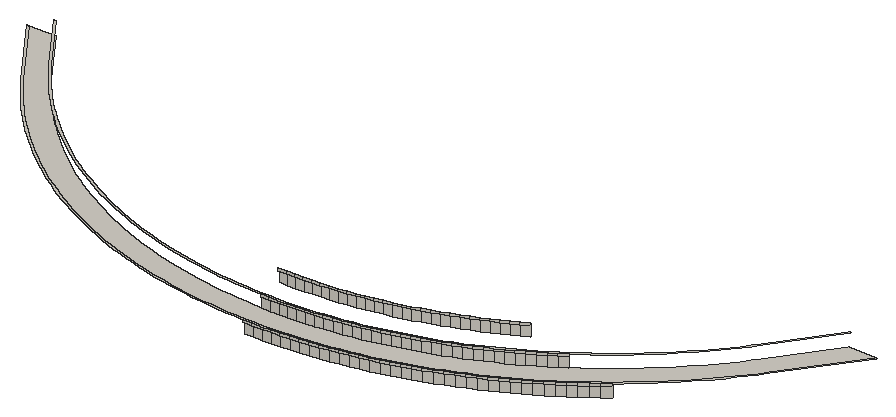
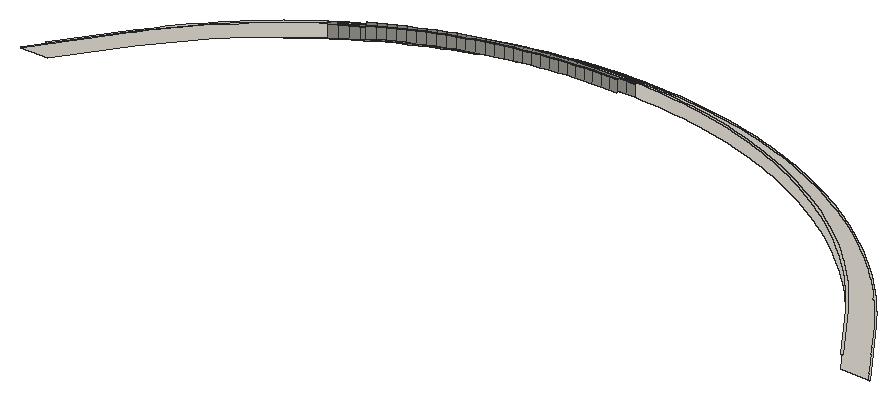
# SketchUp Ruby script. Lengths in inches.
U = 1.inch
M = Sketchup.active_model
def pt(a) = Geom::Point3d.new(a.map { |v| v * U })
def face(e, loops, mat)
  f = e.add_face(loops[0].map { |a| pt(a) })
  loops[1..].each { |l| e.add_face(l.map { |a| pt(a) }).erase! }
  f.material = f.back_material = mat if mat
  f
end
# faces: each face lists its corners as indices into pts; further lists are holes
def faces(e, pts, list, mat = nil) = list.each { |f| face(e, (f[0].is_a?(Array) ? f : [f]).map { |l| l.map { |i| pts[i] } }, mat) }
# xy, xz, yz: faces in a plane at the given z, y or x. An outline is a flat list of corners, or four numbers for a rectangle; further outlines are holes
def ring(l) = l.size == 4 ? [[l[0], l[1]], [l[2], l[1]], [l[2], l[3]], [l[0], l[3]]] : l.each_slice(2).to_a
def flat(e, list, mat, &to3) = list.each { |f| face(e, (f[0].is_a?(Array) ? f : [f]).map { |l| ring(l).map { |u, v| to3.(u, v) } }, mat) }
def xy(e, z, list, mat = nil) = flat(e, list, mat) { |x, y| [x, y, z] }
def xz(e, y, list, mat = nil) = flat(e, list, mat) { |x, z| [x, y, z] }
def yz(e, x, list, mat = nil) = flat(e, list, mat) { |y, z| [x, y, z] }
def lines(e, pts, list) = list.each { |a, b| e.add_line(pt(pts[a]), pt(pts[b])) }
# prism: a flat outline (further loops are holes) pulled along v
def prism(e, loops, v, mat = nil)
  f = face(e, loops, mat); d = Geom::Vector3d.new(v.map { |x| x * U })
  f.pushpull(f.normal.samedirection?(d) ? d.length : -d.length)
end
def box(e, o, s, mat = nil) = prism(e, [[o, [o[0] + s[0], o[1], o[2]], [o[0] + s[0], o[1] + s[1], o[2]], [o[0], o[1] + s[1], o[2]]]], [0, 0, s[2]], mat)
def at(x, y, z, deg = 0) = Geom::Transformation.translation(pt([x, y, z])) * Geom::Transformation.rotation(ORIGIN, Z_AXIS, deg.degrees)
def axes(o, x, y, z) = Geom::Transformation.new([*x, 0, *y, 0, *z, 0, *pt(o).to_a, 1])
def part(name) = M.definitions.add(name)
# library, detail: a bought-in or finely detailed component or shape, given as its bounding box
def library(name, o, s) = part(name).tap { |d| box(d.entities, o, s) }
def detail(e, o, s) = box(e.add_group.entities, o, s)
def put(e, d, t, mat = nil) = e.add_instance(d, t).tap { |i| i.material = mat if mat }
def group(e, t, mat = nil) = e.add_group.tap { |g| g.transformation = t; g.material = mat if mat }.entities
root = M.entities
M.materials.add("Arta-Ceramic-Moonstone-White-24x24-4K").color = [209, 205, 196]
xy(root,6,[[1024.28,78.45,1028.24,78.49,1032.2,78.6,1036.16,78.79,1040.11,79.06,1044.06,79.4,1048,79.82,1051.93,80.31,1055.85,80.88,1059.76,81.52,1063.65,82.24,1067.53,83.03,1071.4,83.9,1075.25,84.84,1079.08,85.85,1082.89,86.94,1086.67,88.1,1090.4375,89.34,1094.18,90.64,1097.89,92.02,1101.58,93.47,1105.24,94.99,1108.87,96.57,1112.47,98.23,1116.03,99.96,1119.5625,101.75,1123.0625,103.61,1126.52,105.54,1129.94,107.54,1133.33,109.6,1136.67,111.72,1139.97,113.91,1143.23,116.16,1146.45,118.47,1149.62,120.85,1152.74,123.28,1155.82,125.78,1158.85,128.33,1161.83,130.94,1164.76,133.61,1167.64,136.33,1170.46,139.11,1173.23,141.94,1175.95,144.82,1178.61,147.76,1181.21,150.75,1183.76,153.78,1186.24,156.87,1188.67,160,1191.04,163.17,1213.38,194.4,1212.72,194.875,1190.38,163.65,1188.02,160.49,1185.6,157.37,1183.13,154.3,1180.59,151.27,1178,148.3,1175.35,145.375,1172.65,142.5,1169.89,139.68,1167.07,136.92,1164.21,134.2,1161.29,131.55,1158.32,128.95,1155.3,126.4,1152.24,123.92,1149.125,121.49,1145.97,119.13,1142.76,116.82,1139.52,114.58,1136.23,112.4,1132.9,110.29,1129.53,108.24,1126.12,106.25,1122.67,104.33,1119.1875,102.47,1115.67,100.6875,1112.12,98.97,1108.54,97.32,1104.92,95.73,1101.28,94.22,1097.6,92.78,1093.9,91.41,1090.18,90.11,1086.43,88.88,1082.66,87.72,1078.86,86.64,1075.05,85.63,1071.21,84.69,1067.36,83.83,1063.5,83.04,1059.62,82.32,1055.72,81.68,1051.82,81.12,1047.9,80.625,1043.98,80.21,1040.05,79.87,1036.11,79.6,1032.17,79.42,1028.23,79.3,1024.28,79.26,1020.34,79.3,1016.39,79.42,1012.45,79.6,1008.51,79.87,1004.58,80.21,1000.66,80.625,996.74,81.12,992.84,81.68,988.94,82.32,985.0625,83.04,981.2,83.83,977.35,84.69,973.51,85.63,969.7,86.64,965.91,87.72,962.13,88.88,958.38,90.11,954.66,91.41,950.96,92.78,947.29,94.22,943.64,95.73,940.03,97.32,936.44,98.97,932.89,100.6875,929.37,102.47,925.89,104.33,922.44,106.25,919.03,108.24,915.66,110.29,912.33,112.4,909.04,114.58,905.8,116.82,902.59,119.13,899.44,121.49,896.32,123.92,893.26,126.4,890.24,128.95,887.27,131.55,884.36,134.2,881.49,136.92,878.68,139.68,875.92,142.5,873.21,145.375,870.5625,148.3,867.97,151.27,865.43,154.3,862.96,157.37,860.54,160.49,858.18,163.65,835.84,194.875,834.84,194.875,857.53,163.17,859.89,160,862.32,156.87,864.81,153.78,867.35,150.75,869.95,147.76,872.61,144.82,875.33,141.94,878.1,139.11,880.92,136.33,883.8,133.61,886.73,130.94,889.71,128.33,892.74,125.78,895.82,123.28,898.94,120.85,902.11,118.47,905.33,116.16,908.59,113.91,911.89,111.72,915.23,109.6,918.62,107.54,922.04,105.54,925.5,103.61,929,101.75,932.53,99.96,936.09,98.23,939.69,96.57,943.32,94.99,946.98,93.47,950.67,92.02,954.38,90.64,958.125,89.34,961.89,88.1,965.68,86.94,969.48,85.85,973.3125,84.84,977.16,83.9,981.03,83.03,984.91,82.24,988.8,81.52,992.71,80.88,996.63,80.31,1000.5625,79.82,1004.5,79.4,1008.45,79.06,1012.4,78.79,1016.36,78.6,1020.32,78.49],[1024.28,79.26,1028.23,79.3,1032.17,79.42,1036.11,79.6,1040.05,79.87,1043.98,80.21,1047.9,80.625,1051.82,81.12,1055.72,81.68,1059.62,82.32,1063.5,83.04,1067.36,83.83,1071.21,84.69,1075.05,85.63,1078.86,86.64,1082.66,87.72,1086.43,88.88,1090.18,90.11,1093.9,91.41,1097.6,92.78,1101.28,94.22,1104.92,95.73,1108.54,97.32,1112.12,98.97,1115.67,100.6875,1119.1875,102.47,1122.67,104.33,1126.12,106.25,1129.53,108.24,1132.9,110.29,1136.23,112.4,1139.52,114.58,1142.76,116.82,1145.97,119.13,1149.125,121.49,1152.24,123.92,1155.3,126.4,1158.32,128.95,1161.29,131.55,1164.21,134.2,1167.07,136.92,1169.89,139.68,1172.65,142.5,1175.35,145.375,1178,148.3,1180.59,151.27,1183.13,154.3,1185.6,157.37,1188.02,160.49,1190.38,163.65,1212.72,194.875,1200.72,194.875,1182.5,169.41,1180.25,166.39,1177.95,163.42,1175.59,160.5,1173.17,157.62,1170.7,154.78,1168.18,152,1165.6,149.26,1162.98,146.58,1160.3,143.94,1157.57,141.36,1154.79,138.83,1151.96,136.35,1149.09,133.93,1146.17,131.56,1143.2,129.25,1140.19,127,1137.14,124.8,1134.05,122.67,1130.92,120.59,1127.74,118.57,1124.53,116.62,1121.29,114.73,1118,112.9,1114.68,111.13,1111.33,109.43,1107.95,107.79,1104.54,106.22,1101.09,104.71,1097.62,103.27,1094.125,101.9,1090.6,100.59,1087.05,99.35,1083.48,98.18,1079.89,97.08,1076.27,96.05,1072.64,95.09,1068.99,94.19,1065.32,93.37,1061.64,92.62,1057.94,91.9375,1054.23,91.33,1050.51,90.79,1046.78,90.32,1043.05,89.92,1039.3,89.6,1035.55,89.35,1031.8,89.17,1028.04,89.06,1024.28,89.02,1020.52,89.06,1016.77,89.17,1013.01,89.35,1009.26,89.6,1005.52,89.92,1001.78,90.32,998.05,90.79,994.33,91.33,990.62,91.9375,986.92,92.62,983.24,93.37,979.57,94.19,975.92,95.09,972.29,96.05,968.68,97.08,965.08,98.18,961.51,99.35,957.96,100.59,954.4375,101.9,950.9375,103.27,947.47,104.71,944.02,106.22,940.61,107.79,937.23,109.43,933.875,111.13,930.56,112.9,927.28,114.73,924.03,116.62,920.82,118.57,917.65,120.59,914.51,122.67,911.42,124.8,908.37,127,905.36,129.25,902.4,131.56,899.48,133.93,896.6,136.35,893.77,138.83,891,141.36,888.27,143.94,885.59,146.58,882.96,149.26,880.38,152,877.86,154.78,875.39,157.62,872.97,160.5,870.61,163.42,868.31,166.39,866.06,169.41,847.84,194.875,835.84,194.875,858.18,163.65,860.54,160.49,862.96,157.37,865.43,154.3,867.97,151.27,870.5625,148.3,873.21,145.375,875.92,142.5,878.68,139.68,881.49,136.92,884.36,134.2,887.27,131.55,890.24,128.95,893.26,126.4,896.32,123.92,899.44,121.49,902.59,119.13,905.8,116.82,909.04,114.58,912.33,112.4,915.66,110.29,919.03,108.24,922.44,106.25,925.89,104.33,929.37,102.47,932.89,100.6875,936.44,98.97,940.03,97.32,943.64,95.73,947.29,94.22,950.96,92.78,954.66,91.41,958.38,90.11,962.13,88.88,965.91,87.72,969.7,86.64,973.51,85.63,977.35,84.69,981.2,83.83,985.0625,83.04,988.94,82.32,992.84,81.68,996.74,81.12,1000.66,80.625,1004.58,80.21,1008.51,79.87,1012.45,79.6,1016.39,79.42,1020.34,79.3]],"Arta-Ceramic-Moonstone-White-24x24-4K")
xy(root,12,[[1024.28,88.21,1028.05,88.25,1031.83,88.36,1035.6,88.54,1039.36,88.79,1043.125,89.11,1046.875,89.51,1050.62,89.98,1054.36,90.52,1058.08,91.14,1061.79,91.82,1065.49,92.58,1069.17,93.4,1072.84,94.3,1076.49,95.26,1080.12,96.3,1083.72,97.41,1087.3125,98.58,1090.875,99.83,1094.41,101.14,1097.93,102.52,1101.41,103.96,1104.87,105.48,1108.3,107.06,1111.7,108.7,1115.06,110.41,1118.39,112.18,1121.6875,114.02,1124.95,115.92,1128.17,117.88,1131.36,119.91,1134.5,121.99,1137.61,124.14,1140.67,126.34,1143.7,128.6,1146.67,130.92,1149.6,133.3,1152.49,135.73,1155.33,138.22,1158.12,140.76,1160.86,143.35,1163.55,146,1166.19,148.7,1168.78,151.45,1171.3125,154.24,1173.79,157.09,1176.22,159.98,1178.59,162.92,1180.9,165.9,1183.15,168.93,1201.71,194.86,1201.05,195.33,1200.72,194.875,1182.5,169.41,1180.25,166.39,1177.95,163.42,1175.59,160.5,1173.17,157.62,1170.7,154.78,1168.18,152,1165.6,149.26,1162.98,146.58,1160.3,143.94,1157.57,141.36,1154.79,138.83,1151.96,136.35,1149.09,133.93,1146.17,131.56,1143.2,129.25,1140.19,127,1137.14,124.8,1134.05,122.67,1130.92,120.59,1127.74,118.57,1124.53,116.62,1121.29,114.73,1118,112.9,1114.68,111.13,1111.33,109.43,1107.95,107.79,1104.54,106.22,1101.09,104.71,1097.62,103.27,1094.125,101.9,1090.6,100.59,1087.05,99.35,1083.48,98.18,1079.89,97.08,1076.27,96.05,1072.64,95.09,1068.99,94.19,1065.32,93.37,1061.64,92.62,1057.94,91.9375,1054.23,91.33,1050.51,90.79,1046.78,90.32,1043.05,89.92,1039.3,89.6,1035.55,89.35,1031.8,89.17,1028.04,89.06,1024.28,89.02,1020.52,89.06,1016.77,89.17,1013.01,89.35,1009.26,89.6,1005.52,89.92,1001.78,90.32,998.05,90.79,994.33,91.33,990.62,91.9375,986.92,92.62,983.24,93.37,979.57,94.19,975.92,95.09,972.29,96.05,968.68,97.08,965.08,98.18,961.51,99.35,957.96,100.59,954.4375,101.9,950.9375,103.27,947.47,104.71,944.02,106.22,940.61,107.79,937.23,109.43,933.875,111.13,930.56,112.9,927.28,114.73,924.03,116.62,920.82,118.57,917.65,120.59,914.51,122.67,911.42,124.8,908.37,127,905.36,129.25,902.4,131.56,899.48,133.93,896.6,136.35,893.77,138.83,891,141.36,888.27,143.94,885.59,146.58,882.96,149.26,880.38,152,877.86,154.78,875.39,157.62,872.97,160.5,870.61,163.42,868.31,166.39,866.06,169.41,847.84,194.875,846.84,194.875,865.41,168.93,867.66,165.9,869.97,162.92,872.34,159.98,874.77,157.09,877.25,154.24,879.78,151.45,882.37,148.7,885.01,146,887.7,143.35,890.44,140.76,893.23,138.22,896.07,135.73,898.96,133.3,901.89,130.92,904.87,128.6,907.89,126.34,910.95,124.14,914.06,121.99,917.2,119.91,920.39,117.88,923.61,115.92,926.875,114.02,930.17,112.18,933.5,110.41,936.87,108.7,940.26,107.06,943.69,105.48,947.15,103.96,950.63,102.52,954.15,101.14,957.6875,99.83,961.25,98.58,964.84,97.41,968.45,96.3,972.07,95.26,975.72,94.3,979.39,93.4,983.07,92.58,986.77,91.82,990.48,91.14,994.21,90.52,997.94,89.98,1001.69,89.51,1005.4375,89.11,1009.2,88.79,1012.96,88.54,1016.73,88.36,1020.51,88.25]],"Arta-Ceramic-Moonstone-White-24x24-4K")
p = [[1024.28,79.26,5],[1024.28,79.26,0],[1028.23,79.3,0],[1028.23,79.3,5],[1032.17,79.42,0],[1032.17,79.42,5],
  [1036.11,79.6,0],[1036.11,79.6,5],[1040.05,79.87,0],[1040.05,79.87,5],[1043.98,80.21,0],[1043.98,80.21,5],
  [1047.9,80.625,0],[1047.9,80.625,5],[1051.82,81.12,0],[1051.82,81.12,5],[1055.72,81.68,0],[1055.72,81.68,5],
  [1059.62,82.32,0],[1059.62,82.32,5],[1063.5,83.04,0],[1063.5,83.04,5],[1067.36,83.83,0],[1067.36,83.83,5],
  [1071.21,84.69,0],[1071.21,84.69,5],[1075.05,85.63,0],[1075.05,85.63,5],[1078.86,86.64,0],[1078.86,86.64,5],
  [1082.66,87.72,0],[1082.66,87.72,5],[1086.43,88.88,0],[1086.43,88.88,5],[1090.18,90.11,0],[1090.18,90.11,5],
  [1093.9,91.41,0],[1093.9,91.41,5],[1097.6,92.78,0],[1097.6,92.78,5],[1101.28,94.22,0],[1101.28,94.22,5],
  [1104.92,95.73,0],[1104.92,95.73,5],[1108.54,97.32,0],[1108.54,97.32,5],[1112.12,98.97,0],[1112.12,98.97,5],
  [1115.67,100.6875,0],[1115.67,100.6875,5],[1119.1875,102.47,0],[1119.1875,102.47,5],[1122.67,104.33,0],[1122.67,104.33,5],
  [1126.12,106.25,0],[1126.12,106.25,5],[1129.53,108.24,0],[1129.53,108.24,5],[1132.9,110.29,0],[1132.9,110.29,5],
  [1136.23,112.4,0],[1136.23,112.4,5],[1139.52,114.58,0],[1139.52,114.58,5],[1142.76,116.82,0],[1142.76,116.82,5],
  [1145.97,119.13,0],[1145.97,119.13,5],[1149.125,121.49,0],[1149.125,121.49,5],[1152.24,123.92,0],[1152.24,123.92,5],
  [1024.28,78.45,6],[1024.28,78.45,5],[1028.24,78.49,5],[1028.24,78.49,6],[1032.2,78.6,5],[1032.2,78.6,6],
  [1036.16,78.79,5],[1036.16,78.79,6],[1040.11,79.06,5],[1040.11,79.06,6],[1044.06,79.4,5],[1044.06,79.4,6],
  [1048,79.82,5],[1048,79.82,6],[1051.93,80.31,5],[1051.93,80.31,6],[1055.85,80.88,5],[1055.85,80.88,6],
  [1059.76,81.52,5],[1059.76,81.52,6],[1063.65,82.24,5],[1063.65,82.24,6],[1067.53,83.03,5],[1067.53,83.03,6],
  [1071.4,83.9,5],[1071.4,83.9,6],[1075.25,84.84,5],[1075.25,84.84,6],[1079.08,85.85,5],[1079.08,85.85,6],
  [1082.89,86.94,5],[1082.89,86.94,6],[1086.67,88.1,5],[1086.67,88.1,6],[1090.4375,89.34,5],[1090.4375,89.34,6],
  [1094.18,90.64,5],[1094.18,90.64,6],[1097.89,92.02,5],[1097.89,92.02,6],[1101.58,93.47,5],[1101.58,93.47,6],
  [1105.24,94.99,5],[1105.24,94.99,6],[1108.87,96.57,5],[1108.87,96.57,6],[1112.47,98.23,5],[1112.47,98.23,6],
  [1116.03,99.96,5],[1116.03,99.96,6],[1119.5625,101.75,5],[1119.5625,101.75,6],[1123.0625,103.61,5],[1123.0625,103.61,6],
  [1126.52,105.54,5],[1126.52,105.54,6],[1129.94,107.54,5],[1129.94,107.54,6],[1133.33,109.6,5],[1133.33,109.6,6],
  [1136.67,111.72,5],[1136.67,111.72,6],[1139.97,113.91,5],[1139.97,113.91,6],[1143.23,116.16,5],[1143.23,116.16,6],
  [1146.45,118.47,5],[1146.45,118.47,6],[1149.62,120.85,5],[1149.62,120.85,6],[1152.74,123.28,5],[1152.74,123.28,6],
  [1024.28,89.02,11],[1024.28,89.02,6],[1028.04,89.06,6],[1028.04,89.06,11],[1031.8,89.17,6],[1031.8,89.17,11],
  [1035.55,89.35,6],[1035.55,89.35,11],[1039.3,89.6,6],[1039.3,89.6,11],[1043.05,89.92,6],[1043.05,89.92,11],
  [1046.78,90.32,6],[1046.78,90.32,11],[1050.51,90.79,6],[1050.51,90.79,11],[1054.23,91.33,6],[1054.23,91.33,11],
  [1057.94,91.9375,6],[1057.94,91.9375,11],[1061.64,92.62,6],[1061.64,92.62,11],[1065.32,93.37,6],[1065.32,93.37,11],
  [1068.99,94.19,6],[1068.99,94.19,11],[1072.64,95.09,6],[1072.64,95.09,11],[1076.27,96.05,6],[1076.27,96.05,11],
  [1079.89,97.08,6],[1079.89,97.08,11],[1083.48,98.18,6],[1083.48,98.18,11],[1087.05,99.35,6],[1087.05,99.35,11],
  [1090.6,100.59,6],[1090.6,100.59,11],[1094.125,101.9,6],[1094.125,101.9,11],[1097.62,103.27,6],[1097.62,103.27,11],
  [1101.09,104.71,6],[1101.09,104.71,11],[1104.54,106.22,6],[1104.54,106.22,11],[1107.95,107.79,6],[1107.95,107.79,11],
  [1111.33,109.43,6],[1111.33,109.43,11],[1114.68,111.13,6],[1114.68,111.13,11],[1118,112.9,6],[1118,112.9,11],
  [1121.29,114.73,6],[1121.29,114.73,11],[1124.53,116.62,6],[1124.53,116.62,11],[1127.74,118.57,6],[1127.74,118.57,11],
  [1130.92,120.59,6],[1130.92,120.59,11],[1134.05,122.67,6],[1134.05,122.67,11],[1024.28,88.21,12],[1024.28,88.21,11],
  [1028.05,88.25,11],[1028.05,88.25,12],[1031.83,88.36,11],[1031.83,88.36,12],[1035.6,88.54,11],[1035.6,88.54,12],
  [1039.36,88.79,11],[1039.36,88.79,12],[1043.125,89.11,11],[1043.125,89.11,12],[1046.875,89.51,11],[1046.875,89.51,12],
  [1050.62,89.98,11],[1050.62,89.98,12],[1054.36,90.52,11],[1054.36,90.52,12],[1058.08,91.14,11],[1058.08,91.14,12],
  [1061.79,91.82,11],[1061.79,91.82,12],[1065.49,92.58,11],[1065.49,92.58,12],[1069.17,93.4,11],[1069.17,93.4,12],
  [1072.84,94.3,11],[1072.84,94.3,12],[1076.49,95.26,11],[1076.49,95.26,12],[1080.12,96.3,11],[1080.12,96.3,12],
  [1083.72,97.41,11],[1083.72,97.41,12],[1087.3125,98.58,11],[1087.3125,98.58,12],[1090.875,99.83,11],[1090.875,99.83,12],
  [1094.41,101.14,11],[1094.41,101.14,12],[1097.93,102.52,11],[1097.93,102.52,12],[1101.41,103.96,11],[1101.41,103.96,12],
  [1104.87,105.48,11],[1104.87,105.48,12],[1108.3,107.06,11],[1108.3,107.06,12],[1111.7,108.7,11],[1111.7,108.7,12],
  [1115.06,110.41,11],[1115.06,110.41,12],[1118.39,112.18,11],[1118.39,112.18,12],[1121.6875,114.02,11],[1121.6875,114.02,12],
  [1124.95,115.92,11],[1124.95,115.92,12],[1128.17,117.88,11],[1128.17,117.88,12],[1131.36,119.91,11],[1131.36,119.91,12],
  [1134.5,121.99,11],[1134.5,121.99,12],[1024.28,98.78,17],[1024.28,98.78,12],[1027.85,98.82,12],[1027.85,98.82,17],
  [1031.42,98.92,12],[1031.42,98.92,17],[1034.99,99.09,12],[1034.99,99.09,17],[1038.55,99.33,12],[1038.55,99.33,17],
  [1042.11,99.64,12],[1042.11,99.64,17],[1045.66,100.02,12],[1045.66,100.02,17],[1049.21,100.46,12],[1049.21,100.46,17],
  [1052.74,100.97,12],[1052.74,100.97,17],[1056.26,101.55,12],[1056.26,101.55,17],[1059.78,102.2,12],[1059.78,102.2,17],
  [1063.28,102.91,12],[1063.28,102.91,17],[1066.76,103.7,12],[1066.76,103.7,17],[1070.23,104.54,12],[1070.23,104.54,17],
  [1073.68,105.46,12],[1073.68,105.46,17],[1077.12,106.4375,12],[1077.12,106.4375,17],[1080.53,107.49,12],[1080.53,107.49,17],
  [1083.92,108.6,12],[1083.92,108.6,17],[1087.3,109.77,12],[1087.3,109.77,17],[1090.64,111.02,12],[1090.64,111.02,17],
  [1093.97,112.32,12],[1093.97,112.32,17],[1097.27,113.69,12],[1097.27,113.69,17],[1100.54,115.12,12],[1100.54,115.12,17],
  [1103.78,116.62,12],[1103.78,116.62,17],[1107,118.17,12],[1107,118.17,17],[1110.18,119.79,12],[1110.18,119.79,17],
  [1113.33,121.47,12],[1113.33,121.47,17],[1116.45,123.21,12],[1116.45,123.21,17],[1024.28,97.97,18],[1024.28,97.97,17],
  [1027.87,98,17],[1027.87,98,18],[1031.45,98.11,17],[1031.45,98.11,18],[1035.04,98.28,17],[1035.04,98.28,18],
  [1038.61,98.52,17],[1038.61,98.52,18],[1042.1875,98.83,17],[1042.1875,98.83,18],[1045.76,99.21,17],[1045.76,99.21,18],
  [1049.3125,99.65,17],[1049.3125,99.65,18],[1052.86,100.17,17],[1052.86,100.17,18],[1056.4,100.75,17],[1056.4,100.75,18],
  [1059.93,101.4,17],[1059.93,101.4,18],[1063.45,102.12,17],[1063.45,102.12,18],[1066.95,102.9,17],[1066.95,102.9,18],
  [1070.43,103.76,17],[1070.43,103.76,18],[1073.9,104.67,17],[1073.9,104.67,18],[1077.35,105.66,17],[1077.35,105.66,18],
  [1080.78,106.71,17],[1080.78,106.71,18],[1084.18,107.83,17],[1084.18,107.83,18],[1087.57,109.01,17],[1087.57,109.01,18],
  [1090.93,110.26,17],[1090.93,110.26,18],[1094.27,111.57,17],[1094.27,111.57,18],[1097.59,112.94,17],[1097.59,112.94,18],
  [1100.87,114.38,17],[1100.87,114.38,18],[1104.13,115.88,17],[1104.13,115.88,18],[1107.36,117.44,17],[1107.36,117.44,18],
  [1110.56,119.07,17],[1110.56,119.07,18],[1113.72,120.75,17],[1113.72,120.75,18],[1116.86,122.5,17],[1116.86,122.5,18]]
faces(root,p,[[0,1,2,3],[3,2,4,5],[5,4,6,7],[7,6,8,9],[9,8,10,11],[11,10,12,13],[13,12,14,15],[15,14,16,17],
  [17,16,18,19],[19,18,20,21],[21,20,22,23],[23,22,24,25],[25,24,26,27],[27,26,28,29],[29,28,30,31],[31,30,32,33],
  [33,32,34,35],[35,34,36,37],[37,36,38,39],[39,38,40,41],[41,40,42,43],[43,42,44,45],[45,44,46,47],[47,46,48,49],
  [49,48,50,51],[51,50,52,53],[53,52,54,55],[55,54,56,57],[57,56,58,59],[59,58,60,61],[61,60,62,63],[63,62,64,65],
  [65,64,66,67],[67,66,68,69],[69,68,70,71],[72,73,74,75],[75,74,76,77],[77,76,78,79],[79,78,80,81],[81,80,82,83],
  [83,82,84,85],[85,84,86,87],[87,86,88,89],[89,88,90,91],[91,90,92,93],[93,92,94,95],[95,94,96,97],[97,96,98,99],
  [99,98,100,101],[101,100,102,103],[103,102,104,105],[105,104,106,107],[107,106,108,109],[109,108,110,111],[111,110,112,113],[113,112,114,115],
  [115,114,116,117],[117,116,118,119],[119,118,120,121],[121,120,122,123],[123,122,124,125],[125,124,126,127],[127,126,128,129],[129,128,130,131],
  [131,130,132,133],[133,132,134,135],[135,134,136,137],[137,136,138,139],[139,138,140,141],[141,140,142,143],[144,145,146,147],[147,146,148,149],
  [149,148,150,151],[151,150,152,153],[153,152,154,155],[155,154,156,157],[157,156,158,159],[159,158,160,161],[161,160,162,163],[163,162,164,165],
  [165,164,166,167],[167,166,168,169],[169,168,170,171],[171,170,172,173],[173,172,174,175],[175,174,176,177],[177,176,178,179],[179,178,180,181],
  [181,180,182,183],[183,182,184,185],[185,184,186,187],[187,186,188,189],[189,188,190,191],[191,190,192,193],[193,192,194,195],[195,194,196,197],
  [197,196,198,199],[199,198,200,201],[201,200,202,203],[203,202,204,205],[205,204,206,207],[208,209,210,211],[211,210,212,213],[213,212,214,215],
  [215,214,216,217],[217,216,218,219],[219,218,220,221],[221,220,222,223],[223,222,224,225],[225,224,226,227],[227,226,228,229],[229,228,230,231],
  [231,230,232,233],[233,232,234,235],[235,234,236,237],[237,236,238,239],[239,238,240,241],[241,240,242,243],[243,242,244,245],[245,244,246,247],
  [247,246,248,249],[249,248,250,251],[251,250,252,253],[253,252,254,255],[255,254,256,257],[257,256,258,259],[259,258,260,261],[261,260,262,263],
  [263,262,264,265],[265,264,266,267],[267,266,268,269],[269,268,270,271],[272,273,274,275],[275,274,276,277],[277,276,278,279],[279,278,280,281],
  [281,280,282,283],[283,282,284,285],[285,284,286,287],[287,286,288,289],[289,288,290,291],[291,290,292,293],[293,292,294,295],[295,294,296,297],
  [297,296,298,299],[299,298,300,301],[301,300,302,303],[303,302,304,305],[305,304,306,307],[307,306,308,309],[309,308,310,311],[311,310,312,313],
  [313,312,314,315],[315,314,316,317],[317,316,318,319],[319,318,320,321],[321,320,322,323],[323,322,324,325],[325,324,326,327],[328,329,330,331],
  [331,330,332,333],[333,332,334,335],[335,334,336,337],[337,336,338,339],[339,338,340,341],[341,340,342,343],[343,342,344,345],[345,344,346,347],
  [347,346,348,349],[349,348,350,351],[351,350,352,353],[353,352,354,355],[355,354,356,357],[357,356,358,359],[359,358,360,361],[361,360,362,363],
  [363,362,364,365],[365,364,366,367],[367,366,368,369],[369,368,370,371],[371,370,372,373],[373,372,374,375],[375,374,376,377],[377,376,378,379],
  [379,378,380,381],[381,380,382,383]],"Arta-Ceramic-Moonstone-White-24x24-4K")
